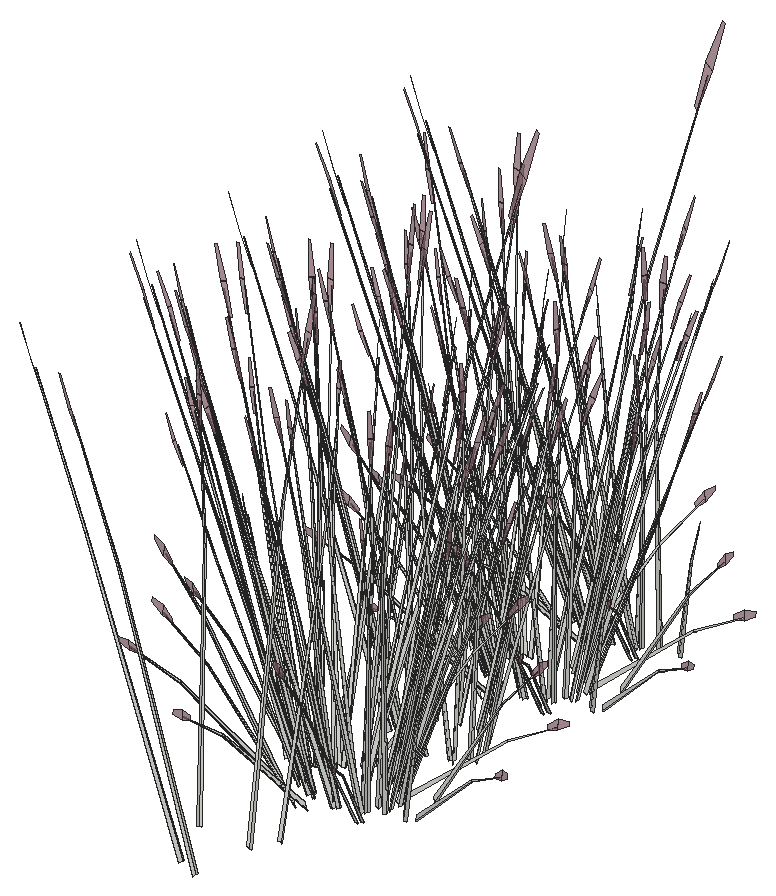
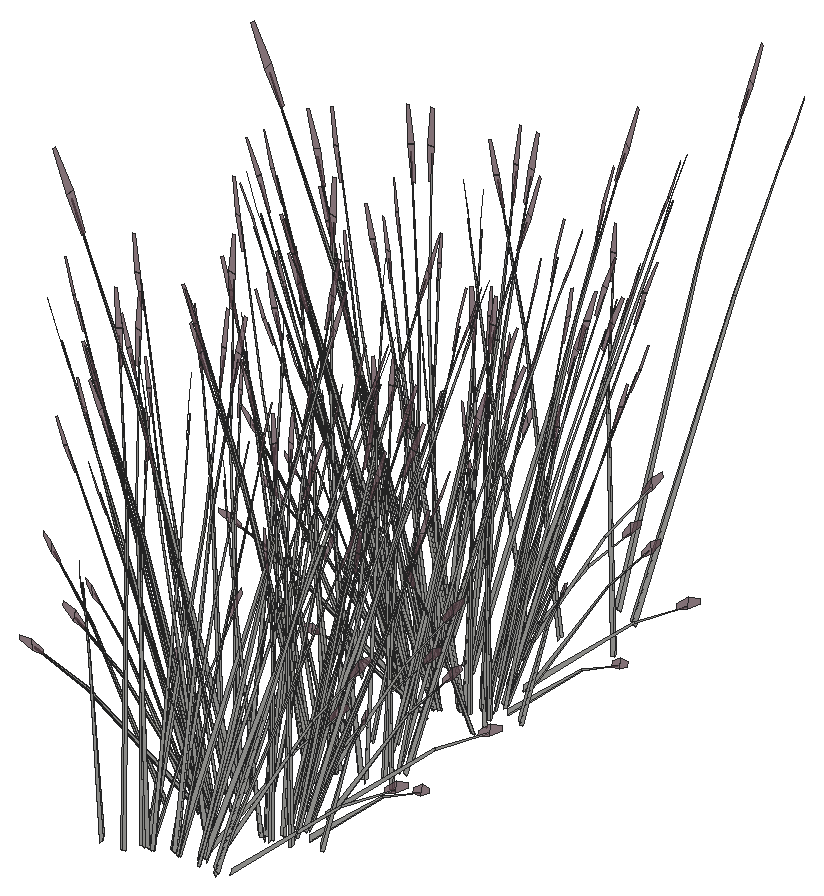
# SketchUp Ruby script. Lengths in inches.
U = 1.inch
M = Sketchup.active_model
def pt(a) = Geom::Point3d.new(a.map { |v| v * U })
def face(e, loops, mat)
  f = e.add_face(loops[0].map { |a| pt(a) })
  loops[1..].each { |l| e.add_face(l.map { |a| pt(a) }).erase! }
  f.material = f.back_material = mat if mat
  f
end
# faces: each face lists its corners as indices into pts; further lists are holes
def faces(e, pts, list, mat = nil) = list.each { |f| face(e, (f[0].is_a?(Array) ? f : [f]).map { |l| l.map { |i| pts[i] } }, mat) }
# xy, xz, yz: faces in a plane at the given z, y or x. An outline is a flat list of corners, or four numbers for a rectangle; further outlines are holes
def ring(l) = l.size == 4 ? [[l[0], l[1]], [l[2], l[1]], [l[2], l[3]], [l[0], l[3]]] : l.each_slice(2).to_a
def flat(e, list, mat, &to3) = list.each { |f| face(e, (f[0].is_a?(Array) ? f : [f]).map { |l| ring(l).map { |u, v| to3.(u, v) } }, mat) }
def xy(e, z, list, mat = nil) = flat(e, list, mat) { |x, y| [x, y, z] }
def xz(e, y, list, mat = nil) = flat(e, list, mat) { |x, z| [x, y, z] }
def yz(e, x, list, mat = nil) = flat(e, list, mat) { |y, z| [x, y, z] }
def lines(e, pts, list) = list.each { |a, b| e.add_line(pt(pts[a]), pt(pts[b])) }
# prism: a flat outline (further loops are holes) pulled along v
def prism(e, loops, v, mat = nil)
  f = face(e, loops, mat); d = Geom::Vector3d.new(v.map { |x| x * U })
  f.pushpull(f.normal.samedirection?(d) ? d.length : -d.length)
end
def box(e, o, s, mat = nil) = prism(e, [[o, [o[0] + s[0], o[1], o[2]], [o[0] + s[0], o[1] + s[1], o[2]], [o[0], o[1] + s[1], o[2]]]], [0, 0, s[2]], mat)
def at(x, y, z, deg = 0) = Geom::Transformation.translation(pt([x, y, z])) * Geom::Transformation.rotation(ORIGIN, Z_AXIS, deg.degrees)
def axes(o, x, y, z) = Geom::Transformation.new([*x, 0, *y, 0, *z, 0, *pt(o).to_a, 1])
def part(name) = M.definitions.add(name)
# library, detail: a bought-in or finely detailed component or shape, given as its bounding box
def library(name, o, s) = part(name).tap { |d| box(d.entities, o, s) }
def detail(e, o, s) = box(e.add_group.entities, o, s)
def put(e, d, t, mat = nil) = e.add_instance(d, t).tap { |i| i.material = mat if mat }
def group(e, t, mat = nil) = e.add_group.tap { |g| g.transformation = t; g.material = mat if mat }.entities
root = M.entities
M.materials.add("LightPink_Translucent").color = [144, 107, 117]
M.materials["LightPink_Translucent"].alpha = 0.75
c1 = part("blade")
p = [[2.15,0.21,22],[0,0.17,0],[0.09,0.45,0],[2.18,0.31,22],[2.29,0.31,22],[0.38,0.45,0],
  [2.48,0.24,33],[2.49,0.24,33],[2.48,0.22,33]]
faces(c1.entities,p,[[0,1,2,3],[4,5,2,3],[6,3,4,7],[8,0,3,6]])
c2 = part("seeds")
p = [[0.3,-0.1,1.38],[-0.01,-0.03,1.59],[-0.01,-0.03,0.03],[0.14,-0.07,-0.07],[0.29,-0.03,3],[0.15,0.01,3.11]]
faces(c2.entities,p,[[0,1,2,3],[1,0,4,5]],"LightPink_Translucent")
c3 = part("blade with seeds")
put(c3.entities,c1,at(0,0,0))
put(c3.entities,c2,axes([2.4,0.25,30.99],[1.5799,-0.05474,1.17369],[-0.12525,1.92788,0.29478],[-0.07173,-0.02425,1.56792]))
put(root,c3,axes([270.87,321.38,127.2],[0.99656,-0.1677,0.53763],[0.17295,0.65785,0.4433],[-0.23438,-0.19388,1.11249]))
put(root,c3,axes([268.85,322.34,127.2],[0.7388,-0.48151,0.53763],[0.63717,0.51135,0.4433],[-0.34662,-0.08882,1.11249]))
put(root,c3,axes([267.17,326.65,127.75],[0.78943,0.17416,-0.06488],[-0.24284,0.53604,-0.29416],[-0.12912,0.08139,0.97024]))
put(root,c3,axes([271.98,333.27,127.73],[-0.13683,-0.09148,1.74944],[-0.91315,0.058,-0.27667],[-0.14574,-0.2188,0.14031]))
put(root,c3,axes([276.09,334.39,127.73],[-0.00864,-0.12985,1.74944],[-0.72937,-0.3753,-0.27667],[0.11277,-0.2275,0.14031]))
put(root,c3,axes([275.89,333.93,127.72],[-0.09085,0.04984,1.77383],[-0.89014,-0.16814,-0.16761],[-0.03222,-0.21748,0.31391]))
put(root,c3,axes([272.74,328.55,127.75],[0.61821,-0.37431,-0.06488],[0.56645,0.40995,-0.29416],[0.03988,0.11616,0.97024]))
put(root,c3,axes([271.05,332.97,127.72],[-0.01669,0.07821,1.77383],[-0.82314,0.28383,-0.16761],[-0.24223,-0.14508,0.31391]))
put(root,c3,axes([270.87,334.36,128.11],[0.99656,-0.1677,0.53763],[0.17295,0.65785,0.4433],[-0.23438,-0.19388,1.11249]))
put(root,c3,axes([271.67,327.17,127.17],[-0.88151,-0.17057,0.53283],[0.30143,-0.56078,0.43934],[0.05297,0.22053,1.10256]))
put(root,c3,axes([273.12,334.48,127.75],[0.88151,0.17057,0.48003],[-0.30143,0.56078,0.3958],[-0.05297,-0.22053,0.9933]))
put(root,c3,axes([273.37,334.68,128.05],[-0.87543,0.30377,-0.1216],[-0.4302,-0.53915,-0.67495],[-0.1155,-0.2272,1.02557]))
put(root,c3,axes([275.19,335.37,128.05],[-0.98321,-0.03233,-0.1216],[0.02687,-0.61208,-0.67495],[0.0683,-0.23574,1.02557]))
put(root,c3,axes([273.35,334.44,127.74],[0.6592,-0.22175,0.0643],[0.32265,0.40436,0.50621],[-0.06366,-0.17825,0.77189]))
put(root,c3,axes([271.09,334.5,127.74],[0.4066,-0.41448,0.0643],[0.57901,0.24131,0.50621],[-0.18719,-0.13288,0.77189]))
put(root,c3,axes([273.11,334.9,128.0625],[-0.2697,0.50175,0.35414],[-0.78684,-0.14635,-0.4572],[-0.07215,-0.20201,0.87481]))
put(root,c3,axes([275.12,335.11,127.75],[0.63704,0.44518,0.48003],[-0.67652,0.38394,0.3958],[0.11751,-0.20886,0.9933]))
put(root,c3,axes([271.28,334.46,128.44],[-0.59706,0.6255,-0.13619],[-0.86465,-0.36036,-0.75594],[-0.30056,-0.17672,1.14864]))
put(root,c3,axes([275.36,335.15,127.74],[0.73517,0.0304,0.0643],[-0.02016,0.45906,0.50621],[0.07693,-0.17585,0.77189]))
put(root,c3,axes([274.81,335.46,128.0625],[-0.60531,0.34352,0.35414],[-0.573,-0.39225,-0.4572],[0.08718,-0.19929,0.87481]))
put(root,c3,axes([268.99,334.28,127.73],[-0.19249,-0.00461,1.74944],[-0.61281,0.46055,-0.27667],[-0.32697,-0.0941,0.14031]))
put(root,c3,axes([276.26,336.57,128.05],[-0.82753,-0.35977,-0.1216],[0.47675,-0.52101,-0.67495],[0.2338,-0.18111,1.02557]))
put(root,c3,axes([271.22,334.98,128.0625],[0.13817,0.52554,0.35414],[-0.78985,0.13877,-0.4572],[-0.21215,-0.1506,0.87481]))
put(root,c3,axes([268.85,335.32,128.11],[0.7388,-0.48151,0.53763],[0.63717,0.51135,0.4433],[-0.34662,-0.08882,1.11249]))
put(root,c3,axes([278.3,336.42,127.72],[-0.11685,-0.00496,1.77383],[-0.48522,-0.53096,-0.16761],[0.19486,-0.17458,0.31391]))
put(root,c3,axes([269.19,335.32,127.74],[0.04505,-0.49615,0.0643],[0.68022,0.0136,0.50621],[-0.26056,-0.05192,0.77189]))
put(root,c3,axes([275.86,336.52,128.0625],[-0.77872,0.09325,0.35414],[-0.20563,-0.53305,-0.4572],[0.22316,-0.14318,0.87481]))
put(root,c3,axes([276.5625,336.4375,127.74],[0.61415,0.2744,0.0643],[-0.35756,0.39076,0.50621],[0.1969,-0.12633,0.77189]))
put(root,c3,axes([276.39,336.32,127.75],[0.22187,0.60049,0.48003],[-0.87033,0.10422,0.3958],[0.25651,-0.14123,0.9933]))
put(root,c3,axes([278.74,337.05,127.73],[0.12414,-0.09938,1.74944],[-0.15889,-0.60963,-0.27667],[0.31148,-0.11559,0.14031]))
put(root,c3,axes([268.25,334.67,127.72],[0.06632,0.06511,1.77383],[-0.31973,0.58531,-0.16761],[-0.32381,0.00424,0.31391]))
put(root,c3,axes([269.65,335.6875,128.0625],[0.50902,0.40851,0.35414],[-0.58122,0.38671,-0.4572],[-0.29531,-0.05884,0.87481]))
put(root,c3,axes([269.51,335.43,128.05],[-0.0479,0.66354,-0.1216],[-0.90696,-0.01814,-0.67495],[-0.3493,-0.04609,1.02557]))
put(root,c3,axes([276.29,337.98,128.05],[-0.45012,-0.59081,-0.1216],[0.79888,-0.29033,-0.67495],[0.33665,-0.07795,1.02557]))
put(root,c3,axes([275.98,337.8,128.0625],[-0.74348,-0.18202,0.35414],[0.21685,-0.53102,-0.4572],[0.29933,-0.04869,0.87481]))
put(root,c3,axes([268.2,336.83,127.75],[0.25275,-0.59491,0.48003],[0.83094,0.20343,0.3958],[-0.32677,0.03575,0.9933]))
put(root,c3,axes([268.14,336.67,127.74],[-0.32857,-0.44488,0.0643],[0.59916,-0.21775,0.50621],[-0.26412,0.04296,0.77189]))
put(root,c3,axes([276.66,337.96,127.74],[0.32857,0.44488,0.0643],[-0.59916,0.21775,0.50621],[0.26412,-0.04296,0.77189]))
put(root,c3,axes([276.59,337.8,127.75],[-0.25275,0.59491,0.48003],[-0.83094,-0.20343,0.3958],[0.32677,-0.03575,0.9933]))
put(root,c3,axes([268.81,336.83,128.0625],[0.74348,0.18202,0.35414],[-0.21685,0.53102,-0.4572],[-0.29933,0.04869,0.87481]))
put(root,c3,axes([278.09,339.73,127.72],[-0.08089,-0.05712,1.77383],[0.17695,-0.61228,-0.16761],[0.31864,-0.03912,0.31391]))
put(root,c3,axes([267.56,337.25,127.73],[-0.14609,0.08471,1.74944],[0.01243,0.61893,-0.27667],[-0.33486,0.08049,0.14031]))
put(root,c3,axes([268.5,336.66,128.05],[0.45012,0.59081,-0.1216],[-0.79888,0.29033,-0.67495],[-0.33665,0.07795,1.02557]))
put(root,c3,axes([275.28,339.2,128.05],[0.0479,-0.66354,-0.1216],[0.90696,0.01814,-0.67495],[0.3493,0.04609,1.02557]))
put(root,c3,axes([275.14,338.94,128.0625],[-0.50902,-0.40851,0.35414],[0.58122,-0.38671,-0.4572],[0.29531,0.05884,0.87481]))
put(root,c3,axes([276.07,338.81,127.73],[0.19191,-0.01103,1.74944],[0.52639,-0.5069,-0.27667],[0.34136,0.06691,0.14031]))
put(root,c3,axes([268.4,338.31,127.75],[-0.22187,-0.60049,0.48003],[0.87033,-0.10422,0.3958],[-0.25651,0.14123,0.9933]))
put(root,c3,axes([268.23,338.19,127.74],[-0.61415,-0.2744,0.0643],[0.35756,-0.39076,0.50621],[-0.1969,0.12633,0.77189]))
put(root,c3,axes([268.93,338.11,128.0625],[0.77872,-0.09325,0.35414],[0.20563,0.53305,-0.4572],[-0.22316,0.14318,0.87481]))
put(root,c3,axes([265.93,337.87,127.72],[0.11417,0.0175,1.77383],[0.35319,0.57649,-0.16761],[-0.23371,0.15131,0.31391]))
put(root,c3,axes([275.61,339.3125,127.74],[-0.04505,0.49615,0.0643],[-0.68022,-0.0136,0.50621],[0.26056,0.05192,0.77189]))
put(root,c3,axes([270.87,344.64,127.42],[0.99656,-0.1677,0.53763],[0.17295,0.65785,0.4433],[-0.23438,-0.19388,1.11249]))
put(root,c3,axes([275.67,339.16,127.75],[-0.65964,0.42992,0.48003],[-0.5689,-0.45657,0.3958],[0.30948,0.0793,0.9933]))
put(root,c3,axes([267.17,339.62,128.66],[0.78943,0.17416,-0.06488],[-0.24284,0.53604,-0.29416],[-0.12912,0.08139,0.97024]))
put(root,c3,axes([273.57,339.65,128.0625],[-0.13817,-0.52554,0.35414],[0.78985,-0.13877,-0.4572],[0.21215,0.1506,0.87481]))
put(root,c3,axes([274.1,336.63,127.49],[-0.77304,-0.33901,1.38283],[0.81626,-0.52782,0.59665],[0.24941,0.31809,1.33663]))
put(root,c3,axes([268.53,338.06,128.05],[0.82753,0.35977,-0.1216],[-0.47675,0.52101,-0.67495],[-0.2338,0.18111,1.02557]))
put(root,c3,axes([273.5,339.92,128.05],[0.53309,-0.55848,-0.1216],[0.77201,0.32175,-0.67495],[0.26836,0.15779,1.02557]))
put(root,c3,axes([273.11,345.17,127.375],[-0.2697,0.50175,0.35414],[-0.78684,-0.14635,-0.4572],[-0.07215,-0.20201,0.87481]))
put(root,c3,axes([275.12,345.38,127.06],[0.63704,0.44518,0.48003],[-0.67652,0.38394,0.3958],[0.11751,-0.20886,0.9933]))
put(root,c3,axes([269.98,339.17,128.0625],[0.60531,-0.34352,0.35414],[0.573,0.39225,-0.4572],[-0.08718,0.19929,0.87481]))
put(root,c3,axes([272.8,340.39,127.72],[0.00265,-0.07899,1.77383],[0.76665,-0.34851,-0.16761],[0.2663,0.12439,0.31391]))
put(root,c3,axes([269.4375,339.48,127.74],[-0.73517,-0.0304,0.0643],[0.02016,-0.45906,0.50621],[-0.07693,0.17585,0.77189]))
put(root,c3,axes([274.81,345.74,127.375],[-0.60531,0.34352,0.35414],[-0.573,-0.39225,-0.4572],[0.08718,-0.19929,0.87481]))
put(root,c3,axes([269.67,339.52,127.75],[-0.63704,-0.44518,0.48003],[0.67652,-0.38394,0.3958],[-0.11751,0.20886,0.9933]))
put(root,c3,axes([271.68,339.74,128.0625],[0.2697,-0.50175,0.35414],[0.78684,0.14635,-0.4572],[0.07215,0.20201,0.87481]))
put(root,c3,axes([273.7,340.13,127.74],[-0.4066,0.41448,0.0643],[-0.57901,-0.24131,0.50621],[0.18719,0.13288,0.77189]))
put(root,c3,axes([272.74,341.53,128.66],[0.61821,-0.37431,-0.06488],[0.56645,0.40995,-0.29416],[0.03988,0.11616,0.97024]))
put(root,c3,axes([273.87,340.01,127.75],[-0.88979,0.14973,0.48003],[-0.15442,-0.58737,0.3958],[0.20926,0.17311,0.9933]))
put(root,c3,axes([271.22,345.25,127.375],[0.13817,0.52554,0.35414],[-0.78985,0.13877,-0.4572],[-0.21215,-0.1506,0.87481]))
put(root,c3,axes([268.85,345.6,127.42],[0.7388,-0.48151,0.53763],[0.63717,0.51135,0.4433],[-0.34662,-0.08882,1.11249]))
put(root,c3,axes([271.4375,340.19,127.74],[-0.6592,0.22175,0.0643],[-0.32265,-0.40436,0.50621],[0.06366,0.17825,0.77189]))
put(root,c3,axes([267.58,339.56,127.73],[-0.02224,0.12912,1.74944],[0.63107,0.44917,-0.27667],[-0.16521,0.21241,0.14031]))
put(root,c3,axes([269.6,339.27,128.41],[0.98321,0.03233,-0.13498],[-0.02687,0.61208,-0.74919],[-0.0683,0.23574,1.13838]))
put(root,c3,axes([271.42,339.95,128.05],[0.87543,-0.30377,-0.1216],[0.4302,0.53915,-0.67495],[0.1155,0.2272,1.02557]))
put(root,c3,axes([271.67,340.15,128.08],[-0.88151,-0.17057,0.53283],[0.30143,-0.56078,0.43934],[0.05297,0.22053,1.10256]))
put(root,c3,axes([275.86,346.8,127.375],[-0.77872,0.09325,0.35414],[-0.20563,-0.53305,-0.4572],[0.22316,-0.14318,0.87481]))
put(root,c3,axes([267.51,340.88,127.72],[0.10149,-0.03939,1.77383],[0.83886,0.26202,-0.16761],[-0.01971,0.21816,0.31391]))
put(root,c3,axes([276.39,346.6,127.06],[0.22187,0.60049,0.48003],[-0.87033,0.10422,0.3958],[0.25651,-0.14123,0.9933]))
put(root,c3,axes([271.21,341.15,127.73],[0.1134,0.10507,1.74944],[0.91515,0.04128,-0.27667],[0.09203,0.23172,0.14031]))
put(root,c3,axes([269.65,345.96,127.375],[0.50902,0.40851,0.35414],[-0.58122,0.38671,-0.4572],[-0.29531,-0.05884,0.87481]))
put(root,c3,axes([275.98,348.07,127.375],[-0.74348,-0.18202,0.35414],[0.21685,-0.53102,-0.4572],[0.29933,-0.04869,0.87481]))
put(root,c3,axes([268.2,347.1,127.06],[0.25275,-0.59491,0.48003],[0.83094,0.20343,0.3958],[-0.32677,0.03575,0.9933]))
put(root,c3,axes([268.81,347.11,127.375],[0.74348,0.18202,0.35414],[-0.21685,0.53102,-0.4572],[-0.29933,0.04869,0.87481]))
put(root,c3,axes([275.14,349.22,127.375],[-0.50902,-0.40851,0.35414],[0.58122,-0.38671,-0.4572],[0.29531,0.05884,0.87481]))
put(root,c3,axes([271.98,354.08,127.36],[-0.13683,-0.09148,1.74944],[-0.91315,0.058,-0.27667],[-0.14574,-0.2188,0.14031]))
put(root,c3,axes([276.09,355.21,127.36],[-0.00864,-0.12985,1.74944],[-0.72937,-0.3753,-0.27667],[0.11277,-0.2275,0.14031]))
put(root,c3,axes([275.89,354.74,127.35],[-0.09085,0.04984,1.77383],[-0.89014,-0.16814,-0.16761],[-0.03222,-0.21748,0.31391]))
put(root,c3,axes([268.93,348.38,127.375],[0.77872,-0.09325,0.35414],[0.20563,0.53305,-0.4572],[-0.22316,0.14318,0.87481]))
put(root,c3,axes([271.05,353.78,127.35],[-0.01669,0.07821,1.77383],[-0.82314,0.28383,-0.16761],[-0.24223,-0.14508,0.31391]))
put(root,c3,axes([270.87,355.17,127.74],[0.99656,-0.1677,0.53763],[0.17295,0.65785,0.4433],[-0.23438,-0.19388,1.11249]))
put(root,c3,axes([273.12,355.29,127.38],[0.88151,0.17057,0.48003],[-0.30143,0.56078,0.3958],[-0.05297,-0.22053,0.9933]))
put(root,c3,axes([267.17,349.9,127.97],[0.78943,0.17416,-0.06488],[-0.24284,0.53604,-0.29416],[-0.12912,0.08139,0.97024]))
put(root,c3,axes([273.35,355.25,127.375],[0.6592,-0.22175,0.0643],[0.32265,0.40436,0.50621],[-0.06366,-0.17825,0.77189]))
put(root,c3,axes([273.57,349.93,127.375],[-0.13817,-0.52554,0.35414],[0.78985,-0.13877,-0.4572],[0.21215,0.1506,0.87481]))
put(root,c3,axes([271.09,355.3125,127.375],[0.4066,-0.41448,0.0643],[0.57901,0.24131,0.50621],[-0.18719,-0.13288,0.77189]))
put(root,c3,axes([269.98,349.45,127.375],[0.60531,-0.34352,0.35414],[0.573,0.39225,-0.4572],[-0.08718,0.19929,0.87481]))
put(root,c3,axes([273.11,355.71,127.7],[-0.2697,0.50175,0.35414],[-0.78684,-0.14635,-0.4572],[-0.07215,-0.20201,0.87481]))
put(root,c3,axes([275.12,355.92,127.38],[0.63704,0.44518,0.48003],[-0.67652,0.38394,0.3958],[0.11751,-0.20886,0.9933]))
put(root,c3,axes([269.67,349.8,127.06],[-0.63704,-0.44518,0.48003],[0.67652,-0.38394,0.3958],[-0.11751,0.20886,0.9933]))
put(root,c3,axes([271.28,355.27,128.08],[-0.59706,0.6255,-0.13619],[-0.86465,-0.36036,-0.75594],[-0.30056,-0.17672,1.14864]))
put(root,c3,axes([275.36,355.96,127.375],[0.73517,0.0304,0.0643],[-0.02016,0.45906,0.50621],[0.07693,-0.17585,0.77189]))
put(root,c3,axes([271.68,350.01,127.375],[0.2697,-0.50175,0.35414],[0.78684,0.14635,-0.4572],[0.07215,0.20201,0.87481]))
put(root,c3,axes([274.81,356.27,127.7],[-0.60531,0.34352,0.35414],[-0.573,-0.39225,-0.4572],[0.08718,-0.19929,0.87481]))
put(root,c3,axes([272.74,351.8,127.97],[0.61821,-0.37431,-0.06488],[0.56645,0.40995,-0.29416],[0.03988,0.11616,0.97024]))
put(root,c3,axes([268.99,355.09,127.36],[-0.19249,-0.00461,1.74944],[-0.61281,0.46055,-0.27667],[-0.32697,-0.0941,0.14031]))
put(root,c3,axes([273.87,350.29,127.06],[-0.88979,0.14973,0.48003],[-0.15442,-0.58737,0.3958],[0.20926,0.17311,0.9933]))
put(root,c3,axes([271.22,355.79,127.7],[0.13817,0.52554,0.35414],[-0.78985,0.13877,-0.4572],[-0.21215,-0.1506,0.87481]))
put(root,c3,axes([268.85,356.13,127.74],[0.7388,-0.48151,0.53763],[0.63717,0.51135,0.4433],[-0.34662,-0.08882,1.11249]))
put(root,c3,axes([278.3,357.23,127.35],[-0.11685,-0.00496,1.77383],[-0.48522,-0.53096,-0.16761],[0.19486,-0.17458,0.31391]))
put(root,c3,axes([271.67,350.42,127.39],[-0.88151,-0.17057,0.53283],[0.30143,-0.56078,0.43934],[0.05297,0.22053,1.10256]))
put(root,c3,axes([269.19,356.13,127.375],[0.04505,-0.49615,0.0643],[0.68022,0.0136,0.50621],[-0.26056,-0.05192,0.77189]))
put(root,c3,axes([275.86,357.33,127.7],[-0.77872,0.09325,0.35414],[-0.20563,-0.53305,-0.4572],[0.22316,-0.14318,0.87481]))
put(root,c3,axes([276.5625,357.25,127.375],[0.61415,0.2744,0.0643],[-0.35756,0.39076,0.50621],[0.1969,-0.12633,0.77189]))
put(root,c3,axes([276.39,357.13,127.38],[0.22187,0.60049,0.48003],[-0.87033,0.10422,0.3958],[0.25651,-0.14123,0.9933]))
put(root,c3,axes([278.74,357.86,127.36],[0.12414,-0.09938,1.74944],[-0.15889,-0.60963,-0.27667],[0.31148,-0.11559,0.14031]))
put(root,c3,axes([268.25,355.48,127.35],[0.06632,0.06511,1.77383],[-0.31973,0.58531,-0.16761],[-0.32381,0.00424,0.31391]))
put(root,c3,axes([269.65,356.5,127.7],[0.50902,0.40851,0.35414],[-0.58122,0.38671,-0.4572],[-0.29531,-0.05884,0.87481]))
put(root,c3,axes([275.98,358.61,127.7],[-0.74348,-0.18202,0.35414],[0.21685,-0.53102,-0.4572],[0.29933,-0.04869,0.87481]))
put(root,c3,axes([268.2,357.64,127.38],[0.25275,-0.59491,0.48003],[0.83094,0.20343,0.3958],[-0.32677,0.03575,0.9933]))
put(root,c3,axes([268.14,357.48,127.375],[-0.32857,-0.44488,0.0643],[0.59916,-0.21775,0.50621],[-0.26412,0.04296,0.77189]))
put(root,c3,axes([276.66,358.77,127.375],[0.32857,0.44488,0.0643],[-0.59916,0.21775,0.50621],[0.26412,-0.04296,0.77189]))
put(root,c3,axes([276.59,358.62,127.38],[-0.25275,0.59491,0.48003],[-0.83094,-0.20343,0.3958],[0.32677,-0.03575,0.9933]))
put(root,c3,axes([268.81,357.65,127.7],[0.74348,0.18202,0.35414],[-0.21685,0.53102,-0.4572],[-0.29933,0.04869,0.87481]))
put(root,c3,axes([278.09,360.54,127.35],[-0.08089,-0.05712,1.77383],[0.17695,-0.61228,-0.16761],[0.31864,-0.03912,0.31391]))
put(root,c3,axes([267.56,358.06,127.36],[-0.14609,0.08471,1.74944],[0.01243,0.61893,-0.27667],[-0.33486,0.08049,0.14031]))
put(root,c3,axes([271.98,363.91,127.39],[-0.13683,-0.09148,1.74944],[-0.91315,0.058,-0.27667],[-0.14574,-0.2188,0.14031]))
put(root,c3,axes([275.14,359.75,127.7],[-0.50902,-0.40851,0.35414],[0.58122,-0.38671,-0.4572],[0.29531,0.05884,0.87481]))
put(root,c3,axes([276.09,365.03,127.39],[-0.00864,-0.12985,1.74944],[-0.72937,-0.3753,-0.27667],[0.11277,-0.2275,0.14031]))
put(root,c3,axes([275.89,364.5625,127.38],[-0.09085,0.04984,1.77383],[-0.89014,-0.16814,-0.16761],[-0.03222,-0.21748,0.31391]))
put(root,c3,axes([276.07,359.62,127.36],[0.19191,-0.01103,1.74944],[0.52639,-0.5069,-0.27667],[0.34136,0.06691,0.14031]))
put(root,c3,axes([268.4,359.12,127.38],[-0.22187,-0.60049,0.48003],[0.87033,-0.10422,0.3958],[-0.25651,0.14123,0.9933]))
put(root,c3,axes([268.23,359,127.375],[-0.61415,-0.2744,0.0643],[0.35756,-0.39076,0.50621],[-0.1969,0.12633,0.77189]))
put(root,c3,axes([271.05,363.61,127.38],[-0.01669,0.07821,1.77383],[-0.82314,0.28383,-0.16761],[-0.24223,-0.14508,0.31391]))
put(root,c3,axes([270.87,364.99,127.77],[0.99656,-0.1677,0.53763],[0.17295,0.65785,0.4433],[-0.23438,-0.19388,1.11249]))
put(root,c3,axes([273.12,365.12,127.41],[0.88151,0.17057,0.48003],[-0.30143,0.56078,0.3958],[-0.05297,-0.22053,0.9933]))
put(root,c3,axes([268.93,358.92,127.7],[0.77872,-0.09325,0.35414],[0.20563,0.53305,-0.4572],[-0.22316,0.14318,0.87481]))
put(root,c3,axes([273.37,365.32,127.71],[-0.87543,0.30377,-0.1216],[-0.4302,-0.53915,-0.67495],[-0.1155,-0.2272,1.02557]))
put(root,c3,axes([275.19,366,127.71],[-0.98321,-0.03233,-0.1216],[0.02687,-0.61208,-0.67495],[0.0683,-0.23574,1.02557]))
put(root,c3,axes([265.93,358.68,127.35],[0.11417,0.0175,1.77383],[0.35319,0.57649,-0.16761],[-0.23371,0.15131,0.31391]))
put(root,c3,axes([273.35,365.07,127.41],[0.6592,-0.22175,0.0643],[0.32265,0.40436,0.50621],[-0.06366,-0.17825,0.77189]))
put(root,c3,axes([275.61,360.125,127.375],[-0.04505,0.49615,0.0643],[-0.68022,-0.0136,0.50621],[0.26056,0.05192,0.77189]))
put(root,c3,axes([275.67,359.97,127.38],[-0.65964,0.42992,0.48003],[-0.5689,-0.45657,0.3958],[0.30948,0.0793,0.9933]))
put(root,c3,axes([271.09,365.14,127.41],[0.4066,-0.41448,0.0643],[0.57901,0.24131,0.50621],[-0.18719,-0.13288,0.77189]))
put(root,c3,axes([267.17,360.43,128.29],[0.78943,0.17416,-0.06488],[-0.24284,0.53604,-0.29416],[-0.12912,0.08139,0.97024]))
put(root,c3,axes([273.57,360.46,127.7],[-0.13817,-0.52554,0.35414],[0.78985,-0.13877,-0.4572],[0.21215,0.1506,0.87481]))
put(root,c3,axes([273.11,365.53,127.73],[-0.2697,0.50175,0.35414],[-0.78684,-0.14635,-0.4572],[-0.07215,-0.20201,0.87481]))
put(root,c3,axes([274.1,357.44,127.12],[-0.77304,-0.33901,1.38283],[0.81626,-0.52782,0.59665],[0.24941,0.31809,1.33663]))
put(root,c3,axes([275.12,365.74,127.41],[0.63704,0.44518,0.48003],[-0.67652,0.38394,0.3958],[0.11751,-0.20886,0.9933]))
put(root,c3,axes([271.28,365.09,128.11],[-0.59706,0.6255,-0.13619],[-0.86465,-0.36036,-0.75594],[-0.30056,-0.17672,1.14864]))
put(root,c3,axes([275.36,365.78,127.41],[0.73517,0.0304,0.0643],[-0.02016,0.45906,0.50621],[0.07693,-0.17585,0.77189]))
put(root,c3,axes([274.81,366.09,127.73],[-0.60531,0.34352,0.35414],[-0.573,-0.39225,-0.4572],[0.08718,-0.19929,0.87481]))
put(root,c3,axes([269.98,359.98,127.7],[0.60531,-0.34352,0.35414],[0.573,0.39225,-0.4572],[-0.08718,0.19929,0.87481]))
put(root,c3,axes([272.8,361.2,127.35],[0.00265,-0.07899,1.77383],[0.76665,-0.34851,-0.16761],[0.2663,0.12439,0.31391]))
put(root,c3,axes([268.99,364.91,127.39],[-0.19249,-0.00461,1.74944],[-0.61281,0.46055,-0.27667],[-0.32697,-0.0941,0.14031]))
put(root,c3,axes([276.26,367.2,127.71],[-0.82753,-0.35977,-0.1216],[0.47675,-0.52101,-0.67495],[0.2338,-0.18111,1.02557]))
put(root,c3,axes([269.4375,360.29,127.375],[-0.73517,-0.0304,0.0643],[0.02016,-0.45906,0.50621],[-0.07693,0.17585,0.77189]))
put(root,c3,axes([269.67,360.34,127.38],[-0.63704,-0.44518,0.48003],[0.67652,-0.38394,0.3958],[-0.11751,0.20886,0.9933]))
put(root,c3,axes([271.68,360.55,127.7],[0.2697,-0.50175,0.35414],[0.78684,0.14635,-0.4572],[0.07215,0.20201,0.87481]))
put(root,c3,axes([271.22,365.61,127.73],[0.13817,0.52554,0.35414],[-0.78985,0.13877,-0.4572],[-0.21215,-0.1506,0.87481]))
put(root,c3,axes([268.85,365.95,127.77],[0.7388,-0.48151,0.53763],[0.63717,0.51135,0.4433],[-0.34662,-0.08882,1.11249]))
put(root,c3,axes([278.3,367.05,127.38],[-0.11685,-0.00496,1.77383],[-0.48522,-0.53096,-0.16761],[0.19486,-0.17458,0.31391]))
put(root,c3,axes([273.7,360.94,127.375],[-0.4066,0.41448,0.0643],[-0.57901,-0.24131,0.50621],[0.18719,0.13288,0.77189]))
put(root,c3,axes([272.74,362.34,128.29],[0.61821,-0.37431,-0.06488],[0.56645,0.40995,-0.29416],[0.03988,0.11616,0.97024]))
put(root,c3,axes([273.87,360.82,127.38],[-0.88979,0.14973,0.48003],[-0.15442,-0.58737,0.3958],[0.20926,0.17311,0.9933]))
put(root,c3,axes([269.19,365.95,127.41],[0.04505,-0.49615,0.0643],[0.68022,0.0136,0.50621],[-0.26056,-0.05192,0.77189]))
